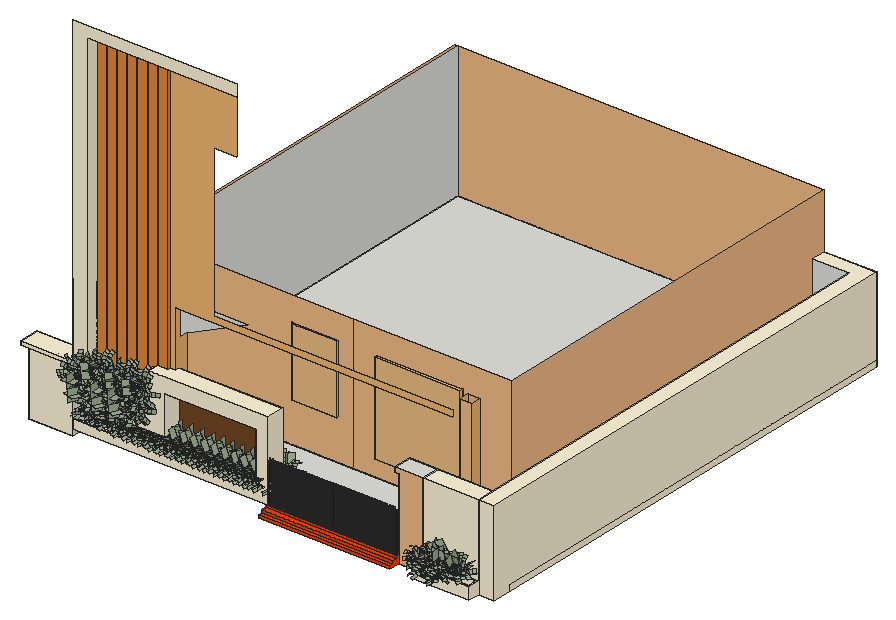
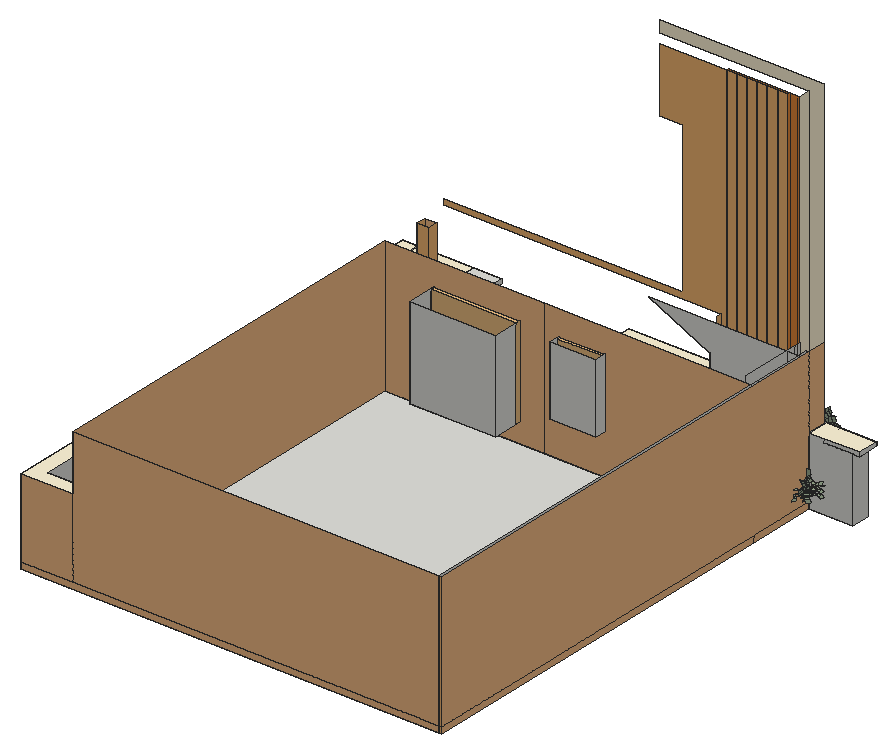
# SketchUp Ruby script. Lengths in inches.
U = 1.inch
M = Sketchup.active_model
def pt(a) = Geom::Point3d.new(a.map { |v| v * U })
def face(e, loops, mat)
  f = e.add_face(loops[0].map { |a| pt(a) })
  loops[1..].each { |l| e.add_face(l.map { |a| pt(a) }).erase! }
  f.material = f.back_material = mat if mat
  f
end
# faces: each face lists its corners as indices into pts; further lists are holes
def faces(e, pts, list, mat = nil) = list.each { |f| face(e, (f[0].is_a?(Array) ? f : [f]).map { |l| l.map { |i| pts[i] } }, mat) }
# xy, xz, yz: faces in a plane at the given z, y or x. An outline is a flat list of corners, or four numbers for a rectangle; further outlines are holes
def ring(l) = l.size == 4 ? [[l[0], l[1]], [l[2], l[1]], [l[2], l[3]], [l[0], l[3]]] : l.each_slice(2).to_a
def flat(e, list, mat, &to3) = list.each { |f| face(e, (f[0].is_a?(Array) ? f : [f]).map { |l| ring(l).map { |u, v| to3.(u, v) } }, mat) }
def xy(e, z, list, mat = nil) = flat(e, list, mat) { |x, y| [x, y, z] }
def xz(e, y, list, mat = nil) = flat(e, list, mat) { |x, z| [x, y, z] }
def yz(e, x, list, mat = nil) = flat(e, list, mat) { |y, z| [x, y, z] }
def lines(e, pts, list) = list.each { |a, b| e.add_line(pt(pts[a]), pt(pts[b])) }
# prism: a flat outline (further loops are holes) pulled along v
def prism(e, loops, v, mat = nil)
  f = face(e, loops, mat); d = Geom::Vector3d.new(v.map { |x| x * U })
  f.pushpull(f.normal.samedirection?(d) ? d.length : -d.length)
end
def box(e, o, s, mat = nil) = prism(e, [[o, [o[0] + s[0], o[1], o[2]], [o[0] + s[0], o[1] + s[1], o[2]], [o[0], o[1] + s[1], o[2]]]], [0, 0, s[2]], mat)
def at(x, y, z, deg = 0) = Geom::Transformation.translation(pt([x, y, z])) * Geom::Transformation.rotation(ORIGIN, Z_AXIS, deg.degrees)
def axes(o, x, y, z) = Geom::Transformation.new([*x, 0, *y, 0, *z, 0, *pt(o).to_a, 1])
def part(name) = M.definitions.add(name)
# library, detail: a bought-in or finely detailed component or shape, given as its bounding box
def library(name, o, s) = part(name).tap { |d| box(d.entities, o, s) }
def detail(e, o, s) = box(e.add_group.entities, o, s)
def put(e, d, t, mat = nil) = e.add_instance(d, t).tap { |i| i.material = mat if mat }
def group(e, t, mat = nil) = e.add_group.tap { |g| g.transformation = t; g.material = mat if mat }.entities
root = M.entities
M.materials.add("[Cladding Siding Tan]").color = [114, 71, 33]
M.materials.add("[Color B05]").color = [255, 63, 0]
M.materials.add("[Color C03]").color = [242, 183, 116]
M.materials.add("[Color C03]1").color = [242, 188, 135]
M.materials.add("[Color D01]").color = [255, 245, 216]
M.materials.add("[Color M08]").color = [30, 30, 30]
M.materials.add("[Wood Bamboo]").color = [226, 136, 59]
M.materials.add("hymenocallis littoralis").color = [156, 172, 146]
c1 = part("Group\#856")
xy(c1.entities,7.38,[[0,0,5.5,15.91]],"hymenocallis littoralis")
p = [[5.5,28.78,0],[5.5,26.79,3.44],[0,26.79,3.44],[0,28.78,0],[0,23.75,6],[5.5,23.75,6],
  [0,15.91,7.38],[5.5,15.91,7.38]]
faces(c1.entities,p,[[0,1,2,3],[4,2,1,5],[6,4,5,7]],"hymenocallis littoralis")
c2 = part("Group\#12")
xy(c2.entities,7.38,[[0,0,5.5,15.91],[0,15.91,5.5,23.87]],"hymenocallis littoralis")
p = [[5.5,31.07,4.3],[5.5,27.74,6.47],[0,27.74,6.47],[0,31.07,4.3],[0,23.87,7.38],[5.5,23.87,7.38]]
faces(c2.entities,p,[[0,1,2,3],[4,2,1,5]],"hymenocallis littoralis")
c3 = part("Group\#857")
xy(c3.entities,7.38,[[0,0,5.6,15.91]],"hymenocallis littoralis")
p = [[5.6,28.78,0],[5.6,26.79,3.44],[0,26.79,3.44],[0,28.78,0],[0,23.75,6],[5.6,23.75,6],
  [0,15.91,7.38],[5.6,15.91,7.38]]
faces(c3.entities,p,[[0,1,2,3],[4,2,1,5],[6,4,5,7]],"hymenocallis littoralis")
c4 = part("Group\#855")
put(c4.entities,c2,axes([6.09,8.57,-0.52],[0.446,0.85617,0.26089],[-0.18444,-0.19731,0.96283],[0.87582,-0.47754,0.0699]))
put(c4.entities,c2,axes([6.29,7.28,-1.71],[0.37058,0.92707,-0.05667],[-0.32382,0.19004,0.99128],[0.87712,-0.32925,0.34964]))
put(c4.entities,c2,axes([11.04,16.14,-0.7],[1,0,0],[0,0.16628,1.02662],[0,-1.18456,0.19186]))
c5 = part("Group\#860")
put(c5.entities,c1,axes([24.57,32.05,-1.76],[0.9552,-0.22102,-0.19681],[0.4036,0.95545,0.88585],[-0.00568,-0.67859,0.7345]))
put(c5.entities,c1,axes([23.95,29.24,-2.4],[0,1,0],[-0.76041,0,0.64945],[0.64945,0,0.76041]))
put(c5.entities,c1,axes([24.22,24.72,-0.48],[-0.70711,0.70711,0],[-0.32757,-0.32757,0.80237],[0.61237,0.61237,0.5]))
put(c5.entities,c2,axes([20.66,37.22,-0.63],[1.12361,0.03262,0.39091],[-0.43499,0.29739,0.78777],[0.09852,-1.27434,0.37535]))
put(c5.entities,c1,axes([28.75,24.45,-2.4],[-1,0,0],[0,-0.76041,0.64945],[0,0.64945,0.76041]))
put(c5.entities,c3,axes([30.4,30.98,-3.7],[0.65676,-0.72002,0.22414],[0.55667,0.66341,0.5],[-0.50871,-0.20361,0.83652]))
put(c5.entities,c3,axes([32.41,29.61,-3.7],[0.04029,-0.97372,0.22414],[0.85287,0.15038,0.5],[-0.52057,0.17102,0.83652]))
put(c5.entities,c1,axes([31.89,25.85,-1.76],[-0.92056,0.33739,-0.19681],[-0.5186,-0.89824,0.88585],[0.08952,0.67268,0.7345]))
put(c5.entities,c1,axes([25.55,34.78,-0.48],[0.86603,0.5,0],[-0.25,0.43301,0.86603],[0.43301,-0.75,0.5]))
put(c5.entities,c3,axes([20.4,16.9375,-8.07],[-0.70711,0.70711,0],[-0.35754,-0.35754,0.65422],[1.3987,1.3987,1.52882]))
put(c5.entities,c1,axes([32.86,34.14,-0.48],[0.76604,-0.64279,0],[0.32139,0.38302,0.86603],[-0.55667,-0.66341,0.5]))
put(c5.entities,c1,axes([27.15,34.7,-0.1],[0.82472,-0.17528,-0.53769],[0.53769,0.53769,0.64945],[0.17528,-0.82472,0.53769]))
put(c5.entities,c1,axes([33.58,28.77,-2.4],[0,-1,0],[0.76041,0,0.64945],[-0.64945,0,0.76041]))
put(c5.entities,c1,axes([26.43,23.87,-2.81],[-0.75126,0.04415,0.65853],[0.53769,-0.53769,0.64945],[0.38276,0.84199,0.3802]))
put(c5.entities,c1,axes([28.78,23.98,-2.4],[-1,0,0],[0,-0.76041,0.64945],[0,0.64945,0.76041]))
put(c5.entities,c1,axes([25.39,25.38,-2.4],[-0.70711,0.70711,0],[-0.53769,-0.53769,0.64945],[0.45923,0.45923,0.76041]))
put(c5.entities,c1,axes([27.32,21.63,-0.1],[-0.45923,0.70711,-0.53769],[-0.76041,0,0.64945],[0.45923,0.70711,0.53769]))
put(c5.entities,c1,axes([25.17,27.625,-1.76],[0.56416,0.80187,-0.19681],[-0.66673,0.66673,0.80532],[0.62659,-0.26057,0.7345]))
put(c5.entities,c3,axes([27.59,27.04,-3.96],[-0.8993,-0.06127,0.43301],[0.2962,-0.8138,0.5],[0.32175,0.57791,0.75]))
put(c5.entities,c3,axes([26.98,24.5,-3.18],[-0.5,0.86603,0],[-0.75,-0.43301,0.5],[0.43301,0.25,0.86603]))
put(c5.entities,c3,axes([24.55,27.74,-3.7],[0.29517,0.92878,0.22414],[-0.85287,0.15038,0.5],[0.43068,-0.33875,0.83652]))
put(c5.entities,c3,axes([24.26,29.8,-3.18],[0.76604,0.64279,0],[-0.47317,0.5639,0.425],[0.32139,-0.38302,0.86603]))
put(c5.entities,c3,axes([25.98,32.46,-3.18],[1,0,0],[0,0.86603,0.5],[0,-0.5,0.86603]))
put(c5.entities,c1,axes([28.78,33.57,-2.4],[1,0,0],[0,0.76041,0.64945],[0,-0.64945,0.76041]))
put(c5.entities,c4,at(14.99,21.38,2.5))
put(c5.entities,c2,axes([34.63,26.34,-1.46],[-0.70089,-0.70877,0.07994],[0.4756,-0.38088,0.79293],[-0.53156,0.59378,0.60405]))
put(c5.entities,c2,axes([28.14,16.92,1.8125],[-1.19719,0.6912,0],[-0.09607,-0.16641,0.94244],[0.68444,1.18549,0.17613]))
put(c5.entities,c2,axes([31.5625,35.84,0.97],[0.66765,-1.1564,0.35779],[0.04445,0.30732,0.91033],[-1.20828,-0.64496,0.17012]))
put(c5.entities,c2,axes([38.94,22.51,0.89],[-0.97932,-0.67164,-0.05202],[0.27787,-0.41401,0.90999],[-0.85985,0.93577,0.32097]))
put(c5.entities,c2,axes([38.44,21.09,1.98],[-1.02864,-0.54856,0.2395],[0.33481,0.06999,0.88388],[-0.77261,1.08328,0.06417]))
put(c5.entities,c3,axes([35.02,30.51,-1.3],[-0.17365,-0.98481,0],[0.60224,-0.10619,0.79122],[-0.7792,0.13739,0.61153]))
put(c5.entities,c3,axes([29.41,22.33,-1.3],[-0.93969,0.34202,0],[-0.20915,-0.57465,0.79122],[0.27061,0.74351,0.61153]))
put(c5.entities,c2,axes([19.64,36,-1.62],[1.18194,0.09546,0.08234],[-0.14377,0.68823,0.76313],[0.21457,-1.1326,0.62386]))
put(c5.entities,c3,axes([24.25,24.14,-1.3],[-0.34202,0.93969,0],[-0.57465,-0.20915,0.79122],[0.74351,0.27061,0.61153]))
put(c5.entities,c3,axes([25.98,34.61,-1.3],[1,0,0],[0,0.61153,0.79122],[0,-0.79122,0.61153]))
put(c5.entities,c3,axes([31.16,34.41,-1.64],[0.56518,-0.80224,-0.19234],[0.73413,0.34233,0.72935],[-0.47639,-0.50772,0.71782]))
put(c5.entities,c3,axes([40.52,26.84,-5.82],[-0.42262,-0.90631,0],[0.48019,-0.22391,0.68552],[-1.43418,0.66877,1.22305]))
put(c5.entities,c1,axes([29.86,38.42,-1.01],[0.89064,-0.37013,0.26413],[-0.03924,0.63286,1.01918],[-0.45353,-0.76487,0.45748]))
put(c5.entities,c1,axes([29.34,22.4,-0.48],[-0.99619,-0.08716,0],[0.04358,-0.4981,0.86603],[-0.07548,0.86273,0.5]))
c6 = part("Group\#859")
put(c6.entities,c1,axes([24.57,32.05,-1.76],[0.9552,-0.22102,-0.19681],[0.4036,0.95545,0.88585],[-0.00568,-0.67859,0.7345]))
put(c6.entities,c1,axes([23.95,29.24,-2.4],[0,1,0],[-0.76041,0,0.64945],[0.64945,0,0.76041]))
put(c6.entities,c1,axes([24.22,24.72,-0.48],[-0.70711,0.70711,0],[-0.32757,-0.32757,0.80237],[0.61237,0.61237,0.5]))
put(c6.entities,c2,axes([22.87,39.97,-0.63],[1.12361,0.03262,0.39091],[-0.43499,0.29739,0.78777],[0.09852,-1.27434,0.37535]))
put(c6.entities,c1,axes([28.75,24.45,-2.4],[-1,0,0],[0,-0.76041,0.64945],[0,0.64945,0.76041]))
put(c6.entities,c3,axes([30.4,30.98,-3.7],[0.65676,-0.72002,0.22414],[0.55667,0.66341,0.5],[-0.50871,-0.20361,0.83652]))
put(c6.entities,c3,axes([32.41,29.61,-3.7],[0.04029,-0.97372,0.22414],[0.85287,0.15038,0.5],[-0.52057,0.17102,0.83652]))
put(c6.entities,c1,axes([31.89,25.85,-1.76],[-0.92056,0.33739,-0.19681],[-0.5186,-0.89824,0.88585],[0.08952,0.67268,0.7345]))
put(c6.entities,c1,axes([25.55,34.78,-0.48],[0.86603,0.5,0],[-0.25,0.43301,0.86603],[0.43301,-0.75,0.5]))
put(c6.entities,c3,axes([20.4,16.9375,-8.07],[-0.70711,0.70711,0],[-0.35754,-0.35754,0.65422],[1.3987,1.3987,1.52882]))
put(c6.entities,c1,axes([32.86,34.14,-0.48],[0.76604,-0.64279,0],[0.32139,0.38302,0.86603],[-0.55667,-0.66341,0.5]))
put(c6.entities,c1,axes([27.15,34.7,-0.1],[0.82472,-0.17528,-0.53769],[0.53769,0.53769,0.64945],[0.17528,-0.82472,0.53769]))
put(c6.entities,c1,axes([33.58,28.77,-2.4],[0,-1,0],[0.76041,0,0.64945],[-0.64945,0,0.76041]))
put(c6.entities,c1,axes([26.43,23.87,-2.81],[-0.75126,0.04415,0.65853],[0.53769,-0.53769,0.64945],[0.38276,0.84199,0.3802]))
put(c6.entities,c1,axes([28.78,23.98,-2.4],[-1,0,0],[0,-0.76041,0.64945],[0,0.64945,0.76041]))
put(c6.entities,c1,axes([25.39,25.38,-2.4],[-0.70711,0.70711,0],[-0.53769,-0.53769,0.64945],[0.45923,0.45923,0.76041]))
put(c6.entities,c1,axes([27.32,21.63,-0.1],[-0.45923,0.70711,-0.53769],[-0.76041,0,0.64945],[0.45923,0.70711,0.53769]))
put(c6.entities,c1,axes([25.17,27.625,-1.76],[0.56416,0.80187,-0.19681],[-0.66673,0.66673,0.80532],[0.62659,-0.26057,0.7345]))
put(c6.entities,c3,axes([27.59,27.04,-3.96],[-0.8993,-0.06127,0.43301],[0.2962,-0.8138,0.5],[0.32175,0.57791,0.75]))
put(c6.entities,c3,axes([33.07,28.9375,-1.86],[-0.5,0.86603,0],[-0.86347,-0.49852,0.1661],[0.11853,0.06843,0.98016]))
put(c6.entities,c3,axes([24.55,27.74,-3.7],[0.29517,0.92878,0.22414],[-0.85287,0.15038,0.5],[0.43068,-0.33875,0.83652]))
put(c6.entities,c3,axes([24.26,29.8,-3.18],[0.76604,0.64279,0],[-0.47317,0.5639,0.425],[0.32139,-0.38302,0.86603]))
put(c6.entities,c3,axes([25.98,32.46,-3.18],[1,0,0],[0,0.86603,0.5],[0,-0.5,0.86603]))
put(c6.entities,c1,axes([28.78,33.57,-2.4],[1,0,0],[0,0.76041,0.64945],[0,-0.64945,0.76041]))
put(c6.entities,c4,at(14.99,21.38,2.5))
put(c6.entities,c2,axes([34.63,26.34,-1.46],[-0.70089,-0.70877,0.07994],[0.4756,-0.38088,0.79293],[-0.53156,0.59378,0.60405]))
put(c6.entities,c2,axes([28.14,16.92,1.8125],[-1.19719,0.6912,0],[-0.09607,-0.16641,0.94244],[0.68444,1.18549,0.17613]))
put(c6.entities,c2,axes([31.5625,35.84,0.97],[0.66765,-1.1564,0.35779],[0.04445,0.30732,0.91033],[-1.20828,-0.64496,0.17012]))
put(c6.entities,c2,axes([38.94,22.51,0.89],[-0.97932,-0.67164,-0.05202],[0.27787,-0.41401,0.90999],[-0.85985,0.93577,0.32097]))
put(c6.entities,c2,axes([38.44,21.09,1.98],[-1.02864,-0.54856,0.2395],[0.33481,0.06999,0.88388],[-0.77261,1.08328,0.06417]))
put(c6.entities,c3,axes([35.02,30.51,-1.3],[-0.17365,-0.98481,0],[0.60224,-0.10619,0.79122],[-0.7792,0.13739,0.61153]))
put(c6.entities,c3,axes([29.41,22.33,-1.3],[-0.93969,0.34202,0],[-0.20915,-0.57465,0.79122],[0.27061,0.74351,0.61153]))
put(c6.entities,c2,axes([19.64,36,-1.62],[1.18194,0.09546,0.08234],[-0.14377,0.68823,0.76313],[0.21457,-1.1326,0.62386]))
put(c6.entities,c3,axes([24.25,24.14,-1.3],[-0.34202,0.93969,0],[-0.57465,-0.20915,0.79122],[0.74351,0.27061,0.61153]))
put(c6.entities,c3,axes([25.98,34.61,-1.3],[1,0,0],[0,0.61153,0.79122],[0,-0.79122,0.61153]))
put(c6.entities,c3,axes([31.16,34.41,-1.64],[0.56518,-0.80224,-0.19234],[0.73413,0.34233,0.72935],[-0.47639,-0.50772,0.71782]))
put(c6.entities,c3,axes([40.52,26.84,-5.82],[-0.42262,-0.90631,0],[0.48019,-0.22391,0.68552],[-1.43418,0.66877,1.22305]))
put(c6.entities,c1,axes([29.86,38.42,-1.01],[0.89064,-0.37013,0.26413],[-0.03924,0.63286,1.01918],[-0.45353,-0.76487,0.45748]))
put(c6.entities,c1,axes([29.34,22.4,-0.48],[-0.99619,-0.08716,0],[0.04358,-0.4981,0.86603],[-0.07548,0.86273,0.5]))
put(c6.entities,c3,axes([25.22,28.39,-0.16],[0.48481,0.87462,0],[-0.87203,0.48338,0.1661],[0.11971,-0.06635,0.98016]))
put(c6.entities,c3,axes([24.56,24.29,-4.78],[0.48481,0.87462,0],[-0.87203,0.48338,0.1661],[0.11971,-0.06635,0.98016]))
put(c6.entities,c3,axes([23.9375,27.06,-4.78],[0.99753,0.07018,0],[-0.06998,0.99459,0.1661],[0.00961,-0.13653,0.98016]))
put(c6.entities,c3,axes([25.92,29.09,-4.78],[0.6025,-0.79812,0],[0.79576,0.60072,0.1661],[-0.10924,-0.08246,0.98016]))
put(c6.entities,c3,axes([28.7,28.53,-4.78],[-0.34082,-0.94013,0],[0.93735,-0.33981,0.1661],[-0.12867,0.04665,0.98016]))
c7 = part("Group\#858")
xz(c7.entities,10.07,[[9.07,0,10.07,31.01],[0,31.01,0,45.12,20.13,45.12,20.13,31.01,10.07,31.01,10.07,32.58,9.07,32.58,9.07,31.01]],"hymenocallis littoralis")
yz(c7.entities,10.07,[[0,31.01,20.13,45.12]],"hymenocallis littoralis")
p = [[9.57,9.2,0],[10.07,10.07,0],[10.07,10.07,31.01],[10.07,10.07,32.58],[9.57,9.2,32.58]]
faces(c7.entities,p,[[0,1,2,3,4]],"hymenocallis littoralis")
c8 = part("cây lá nắng")
put(c8.entities,c5,axes([49.26,-2.75,0],[0.63109,0.63109,0],[-0.63109,0.63109,0],[0,0,0.935]))
put(c8.entities,c6,axes([26.6,-8.68,0],[0.63109,0.63109,0],[-0.63109,0.63109,0],[0,0,0.935]))
put(c8.entities,c7,axes([29.71,14.29,6.94],[0.425,0.73612,0],[-0.6771,0.39092,-0.33349],[-0.26859,0.15507,0.72712]))
put(c8.entities,c7,axes([42.0625,26.12,6.94],[0.85,0,0],[0,0.78185,-0.33349],[0,0.33349,0.78185]))
put(c8.entities,c5,axes([7.3125,23.0625,0],[0.8925,0,0],[0,0.8925,0],[0,0,0.935]))
put(c8.entities,c7,axes([24.4375,40.23,2.05],[0.85,0,0],[0,0.85,0],[0,0,0.85]))
c9 = part("Planting+101")
put(c9.entities,c8,axes([21.34,32.96,-4.59],[0,-0.71,0],[-0.71,0,0],[0,0,0.71]))
c10 = part("Group\#428")
prism(c10.entities,[[[0,1.97,0],[0,1.97,1.18],[0,0,1.18],[0,0,0]],[[0,1.92,1.13],[0,1.92,0.05],[0,0.05,0.05],[0,0.05,1.13]]],[98.43,0,0])
c11 = part("Group\#430")
xy(c11.entities,0,[[0.3,0,0.22,0.01,0.15,0.04,0.09,0.09,0.04,0.15,0.01,0.22,0,0.3,0.3,0.3],[0.3,0,0.3,0.3,0.59,0.3,0.58,0.22,0.55,0.15,0.5,0.09,0.44,0.04,0.37,0.01],[0,0.3,0.01,0.37,0.04,0.44,0.09,0.5,0.15,0.55,0.22,0.58,0.3,0.59,0.3,0.3],[0.3,0.3,0.3,0.59,0.37,0.58,0.44,0.55,0.5,0.5,0.55,0.44,0.58,0.37,0.59,0.3]])
xy(c11.entities,39.37,[[0.3,0,0.37,0.01,0.44,0.04,0.5,0.09,0.55,0.15,0.58,0.22,0.59,0.3,0.58,0.37,0.55,0.44,0.5,0.5,0.44,0.55,0.37,0.58,0.3,0.59,0.22,0.58,0.15,0.55,0.09,0.5,0.04,0.44,0.01,0.37,0,0.3,0.01,0.22,0.04,0.15,0.09,0.09,0.15,0.04,0.22,0.01]])
p = [[0.09,0.09,0],[0.15,0.04,0],[0.15,0.04,39.37],[0.09,0.09,39.37],[0.22,0.01,0],[0.22,0.01,39.37],
  [0.3,0,0],[0.3,0,39.37],[0.37,0.01,0],[0.37,0.01,39.37],[0.44,0.04,0],[0.44,0.04,39.37],
  [0.5,0.09,0],[0.5,0.09,39.37],[0.01,0.22,0],[0.04,0.15,0],[0.04,0.15,39.37],[0.01,0.22,39.37],
  [0.55,0.15,0],[0.55,0.15,39.37],[0.58,0.22,0],[0.58,0.22,39.37],[0,0.3,0],[0,0.3,39.37],
  [0.59,0.3,0],[0.59,0.3,39.37],[0.01,0.37,0],[0.01,0.37,39.37],[0.58,0.37,0],[0.58,0.37,39.37],
  [0.09,0.5,0],[0.04,0.44,0],[0.04,0.44,39.37],[0.09,0.5,39.37],[0.55,0.44,0],[0.5,0.5,0],
  [0.5,0.5,39.37],[0.55,0.44,39.37],[0.15,0.55,0],[0.15,0.55,39.37],[0.44,0.55,0],[0.44,0.55,39.37],
  [0.22,0.58,0],[0.22,0.58,39.37],[0.3,0.59,0],[0.3,0.59,39.37],[0.37,0.58,0],[0.37,0.58,39.37]]
faces(c11.entities,p,[[0,1,2,3],[1,4,5,2],[4,6,7,5],[6,8,9,7],[8,10,11,9],[10,12,13,11],[14,15,16,17],[15,0,3,16],
  [12,18,19,13],[18,20,21,19],[22,14,17,23],[20,24,25,21],[26,22,23,27],[24,28,29,25],[30,31,32,33],[31,26,27,32],
  [34,35,36,37],[28,34,37,29],[38,30,33,39],[35,40,41,36],[42,38,39,43],[44,42,43,45],[46,44,45,47],[40,46,47,41]])
c12 = part("Group\#429")
prism(c12.entities,[[[0.01,0.22,35.83],[0,0.3,35.83],[0.01,0.37,35.83],[0.04,0.44,35.83],[0.09,0.5,35.83],[0.15,0.55,35.83],[0.22,0.58,35.83],[0.3,0.59,35.83],[0.37,0.58,35.83],[0.44,0.55,35.83],[0.5,0.5,35.83],[0.55,0.44,35.83],[0.58,0.37,35.83],[0.59,0.3,35.83],[0.58,0.22,35.83],[0.55,0.15,35.83],[0.5,0.09,35.83],[0.44,0.04,35.83],[0.37,0.01,35.83],[0.3,0,35.83],[0.22,0.01,35.83],[0.15,0.04,35.83],[0.09,0.09,35.83],[0.04,0.15,35.83]]],[0,0,3.54])
c13 = part("Picket railing panel")
g1 = group(c13.entities,at(0,0,0))
put(g1,c10,axes([0,0,39.76],[1,0,0],[0,0,-1],[0,1,0]),"[Color M08]")
put(g1,c10,axes([0,0,1.97],[1,0,0],[0,0,-1],[0,1,0]),"[Color M08]")
put(g1,c10,axes([98.43,0,37.8],[0,0,-0.364],[-1,0,0],[0,1,0]),"[Color M08]")
put(g1,c10,axes([1.97,0,37.8],[0,0,-0.364],[-1,0,0],[0,1,0]),"[Color M08]")
g2 = group(c13.entities,at(1.67,0.3,1.97))
put(g2,c11,at(78.74,0,0),"[Color M08]")
put(g2,c11,at(90.55,0,0),"[Color M08]")
put(g2,c11,at(82.68,0,0),"[Color M08]")
put(g2,c11,at(86.61,0,0),"[Color M08]")
put(g2,c11,at(66.93,0,0),"[Color M08]")
put(g2,c11,at(11.8125,0,0),"[Color M08]")
put(g2,c11,at(15.75,0,0),"[Color M08]")
put(g2,c11,at(47.24,0,0),"[Color M08]")
put(g2,c11,at(59.06,0,0),"[Color M08]")
put(g2,c12,at(0,0,0),"[Color M08]")
put(g2,c11,at(39.37,0,0),"[Color M08]")
put(g2,c11,at(62.99,0,0),"[Color M08]")
put(g2,c11,at(55.12,0,0),"[Color M08]")
put(g2,c11,at(19.69,0,0),"[Color M08]")
put(g2,c11,at(35.43,0,0),"[Color M08]")
put(g2,c11,at(7.875,0,0),"[Color M08]")
put(g2,c11,at(23.62,0,0),"[Color M08]")
put(g2,c11,at(31.5,0,0),"[Color M08]")
put(g2,c11,at(43.31,0,0),"[Color M08]")
put(g2,c11,at(27.56,0,0),"[Color M08]")
put(g2,c11,at(3.9375,0,0),"[Color M08]")
put(g2,c11,at(51.18,0,0),"[Color M08]")
put(g2,c11,at(70.87,0,0),"[Color M08]")
put(g2,c11,at(74.8,0,0),"[Color M08]")
put(g2,c12,at(94.49,0,0),"[Color M08]")
c14 = library("Group\#5",[0,0,0],[84,7.18,89.375])
c15 = part("Group\#3")
yz(c15.entities,10,[[0,0,3,309.43]])
g3 = group(c15.entities,at(0,0,0))
xz(g3,0,[[0,0,10,309.43]])
c16 = library("French glass door with glass lintels",[-8.63,0,-6],[91.05,103.25,8])
c17 = library("0bf58b33-bf0e-48eb-9a0e-7b561c723b43",[30.51,1.97,38.58],[7.49,3.24,2.84])
c18 = library("53c5b651-04ed-452e-9df6-41195152b95b",[21.06,1.97,38.58],[7.48,3.24,2.84])
xy(root,0,[[241.3125,20.4,241.3125,49.9,52.3125,49.9,52.3125,117.47,412.3125,117.47,412.3125,49.9,370.28,49.9,370.28,20.4],[393.97,20.4,448.3125,49.9],[6.375,31.9,49.3125,49.9],[370.28,31.9,393.97,49.9],[448.3125,31.9,463.8125,49.9],
  [49.3125,49.9,52.3125,117.47],[412.3125,49.9,412.3125,117.47,52.3125,117.47,52.3125,501.47,463.8125,501.47,463.8125,49.9],[49.3125,117.47,52.3125,501.47]])
xy(root,2.66,[[241.3125,20.4,370.28,24.71]],"[Color B05]")
xy(root,4.375,[[395.18,21.61,447.1,30.69]],"[Color D01]")
xy(root,5.3125,[[241.3125,24.71,370.28,29.52]],"[Color B05]")
xy(root,6,[[49.3125,31.9,241.3125,49.9],[[241.3125,31.9,370.28,31.9,370.28,49.9,448.3125,49.9,448.3125,486.84,412.3125,486.84,412.3125,117.47,52.3125,117.47,52.3125,109.47,63.88,109.47,63.88,59.47,229.04,59.47,229.04,49.9,241.3125,49.9],[399.28,70.78,410.47,80.47]],[49.3125,49.9,52.3125,59.47],[52.3125,49.9,63.88,59.47],[63.88,49.9,139.52,59.47],
  [139.52,49.9,199.52,59.47],[199.52,49.9,229.04,59.47],[448.3125,49.9,463.8125,49.9,463.8125,501.47,412.3125,501.47,412.3125,486.84,448.3125,486.84],[49.3125,59.47,52.3125,109.47],[52.3125,59.47,63.88,109.47],
  [49.3125,109.47,52.3125,117.47],[49.3125,117.47,52.3125,501.47],[52.3125,117.47,412.3125,501.47]])
xy(root,7.3125,[[241.3125,29.52,370.28,31.9]],"[Color B05]")
xy(root,7.8,[[52.05,34.64,226.3,47.16]])
xy(root,12,[[[393.97,20.4,448.3125,31.9],[395.18,21.61,447.1,30.69]]],"[Color D01]")
xy(root,14.3,[[[49.3125,31.9,229.04,49.9],[52.05,34.64,226.3,47.16]]],"[Color D01]")
xy(root,24.625,[[280.3125,117.47,364.3125,146.78]])
xy(root,30.5625,[[49.3125,31.9,139.52,49.9]])
xy(root,45.57,[[63.88,42.9,73.88,42.9,73.88,45.9,123.75,45.9,123.75,49.9,63.88,49.9]])
xy(root,45.57,[[63.88,31.9,123.75,31.9,123.75,45.9,73.88,45.9,73.88,42.9,63.88,42.9]],"[Color D01]")
xy(root,46.125,[[196.3125,117.47,241.3125,128.9]])
xy(root,63.39,[[0,29.15,34.8125,31.9],[34.8125,29.15,49.3125,31.9],[0,31.9,6.375,49.9],[6.375,31.9,34.8125,49.9]])
xy(root,67.02,[[0,29.15,49.3125,49.9]],"[Color D01]")
xy(root,68.78,[[139.52,31.9,229.04,49.9],[139.52,49.9,229.04,59.47]])
xy(root,79.13,[[366.09,31.9,370.28,49.9]])
xy(root,83.44,[[366.09,31.9,393.97,49.9],[123.75,45.9,139.52,49.9]])
xy(root,83.44,[[123.75,31.9,241.3125,31.9,241.3125,49.9,139.52,49.9,139.52,45.9,123.75,45.9],[393.97,31.9,448.3125,49.9],[448.3125,31.9,463.8125,31.9,463.8125,501.47,412.3125,501.47,412.3125,486.84,448.3125,486.84]],"[Color D01]")
xz(root,20.4,[[241.3125,0,370.28,2.66]],"[Color B05]")
xz(root,20.4,[[393.97,0,448.3125,12]],"[Color D01]")
xz(root,21.61,[[395.18,4.375,447.1,12]],"[Color D01]")
xz(root,24.71,[[241.3125,2.66,370.28,5.3125]],"[Color B05]")
xz(root,29.15,[[0,63.39,49.3125,67.02]],"[Color D01]")
xz(root,29.52,[[241.3125,5.3125,370.28,7.3125]],"[Color B05]")
xz(root,30.69,[[395.18,4.375,447.1,12]],"[Color D01]")
xz(root,31.9,[[241.3125,6,370.28,7.3125]])
xz(root,31.9,[[370.28,0,393.97,0,393.97,83.44,366.09,83.44,366.09,79.13,370.28,79.13]],"[Color C03]1")
xz(root,31.9,[[6.375,0,49.3125,63.39],[448.3125,0,463.8125,83.44],[49.3125,6,241.3125,6,241.3125,83.44,123.75,83.44,123.75,45.57,63.88,45.57,63.88,354.99,210.46,354.99,210.46,366,49.3125,366,49.3125,30.5625,139.52,30.5625,139.52,68.78,229.04,68.78,229.04,14.3,49.3125,14.3],[393.97,12,448.3125,83.44]],"[Color D01]")
xz(root,34.64,[[52.05,7.8,226.3,14.3]])
xz(root,45.9,[[73.88,45.57,123.75,45.57,123.75,83.44,139.52,83.44,139.52,138,412.3125,138,412.3125,144,177.125,144,177.125,291.78,199.52,291.78,199.52,354.99,73.88,354.99]],"[Color C03]")
xz(root,47.16,[[52.05,7.8,52.3125,14.3],[52.3125,7.8,63.88,14.3],[63.88,7.8,226.3,14.3]])
xz(root,49.9,[[6.375,0,6.375,63.39,34.8125,63.39,34.8125,67.02,49.3125,67.02,49.3125,0],[49.3125,0,52.3125,6],[370.28,0,393.97,6],[393.97,0,448.3125,6],[448.3125,0,463.8125,6],
  [49.3125,6,52.3125,14.3],[52.3125,6,63.88,14.3],[63.88,6,229.04,14.3],[229.04,6,229.04,68.78,139.52,68.78,139.52,83.44,241.3125,83.44,241.3125,6],[370.28,6,370.28,79.13,366.09,79.13,366.09,83.44,393.97,83.44,393.97,6],
  [393.97,6,448.3125,83.44],[49.3125,30.5625,52.3125,138],[63.88,30.5625,123.75,45.57],[123.75,30.5625,139.52,83.44],[0,63.39,34.8125,67.02]])
xz(root,49.9,[[49.3125,14.3,52.3125,30.5625],[52.3125,14.3,63.88,30.5625],[63.88,14.3,229.04,14.3,229.04,68.78,139.52,68.78,139.52,30.5625,63.88,30.5625]],"[Cladding Siding Tan]")
xz(root,49.9,[[52.3125,0,241.3125,6]],"[Color D01]")
xz(root,59.47,[[52.3125,6,52.3125,138,199.52,138,139.52,109.96,139.52,68.78,229.04,68.78,229.04,6]])
xz(root,70.78,[[399.28,6,410.47,138]],"[Color C03]1")
xz(root,80.47,[[399.28,6,410.47,138]],"[Color C03]")
xz(root,117.47,[[49.3125,0,52.3125,6],[52.3125,0,412.3125,6]])
xz(root,117.47,[[[52.3125,6,256.62,138],[196.3125,46.125,241.3125,114]],[[256.62,6,412.3125,138],[280.3125,24.625,364.3125,114]]],"[Color C03]1")
xz(root,128.9,[[196.3125,46.125,241.3125,114]])
xz(root,146.78,[[280.3125,24.625,364.3125,114]])
xz(root,486.84,[[412.3125,6,448.3125,83.44]])
xz(root,501.47,[[49.3125,0,52.3125,6],[49.3125,6,52.3125,138]],"[Color C03]")
xz(root,501.47,[[52.3125,0,463.8125,6],[52.3125,6,412.3125,138],[412.3125,6,463.8125,83.44]],"[Color C03]1")
yz(root,0,[[29.15,63.39,49.9,67.02]])
yz(root,6.375,[[31.9,0,49.9,63.39]])
yz(root,49.3125,[[31.9,0,49.9,6],[31.9,6,49.9,14.3],[31.9,14.3,49.9,30.5625],[31.9,30.5625,49.9,67.02],[29.15,63.39,31.9,67.02]])
yz(root,49.3125,[[49.9,0,117.47,6],[117.47,0,501.47,6],[49.9,6,501.47,138],[31.9,67.02,49.9,138]],"[Color C03]1")
yz(root,52.05,[[34.64,7.8,47.16,14.3]])
yz(root,52.3125,[[49.9,0,117.47,6],[117.47,0,501.47,6],[49.9,6,59.47,138],[59.47,6,109.47,138],[109.47,6,117.47,138],
  [117.47,6,501.47,138]])
yz(root,63.88,[[49.9,6,109.47,138],[42.9,45.57,49.9,138]])
yz(root,63.88,[[31.9,45.57,42.9,354.99]],"[Color D01]")
yz(root,123.75,[[31.9,45.57,45.9,83.44],[45.9,45.57,49.9,83.44]])
yz(root,139.52,[[49.9,68.78,59.47,68.78,59.47,109.96,50.65,109.96,50.65,138,45.9,138,45.9,83.44,49.9,83.44]],"[Color C03]")
yz(root,139.52,[[31.9,30.5625,49.9,68.78]],"[Color D01]")
yz(root,196.3125,[[117.47,46.125,128.9,114]])
yz(root,226.3,[[34.64,7.8,47.16,14.3]])
yz(root,229.04,[[49.9,6,59.47,68.78]])
yz(root,229.04,[[31.9,14.3,49.9,68.78]],"[Color D01]")
yz(root,241.3125,[[117.47,46.125,128.9,114]])
yz(root,241.3125,[[20.4,0,20.4,2.66,24.71,2.66,24.71,5.3125,29.52,5.3125,29.52,7.3125,31.9,7.3125,31.9,6,49.9,6,49.9,0]],"[Color B05]")
yz(root,241.3125,[[31.9,6,49.9,83.44]],"[Color D01]")
yz(root,280.3125,[[117.47,24.625,146.78,114]])
yz(root,364.3125,[[117.47,24.625,146.78,114]])
yz(root,366.09,[[31.9,79.13,49.9,83.44]])
yz(root,370.28,[[31.9,0,49.9,6],[31.9,6,49.9,79.13]])
yz(root,370.28,[[20.4,0,31.9,0,31.9,7.3125,29.52,7.3125,29.52,5.3125,24.71,5.3125,24.71,2.66,20.4,2.66]],"[Color B05]")
yz(root,393.97,[[31.9,0,49.9,83.44]])
yz(root,393.97,[[20.4,0,31.9,12]],"[Color D01]")
yz(root,395.18,[[21.61,4.375,30.69,12]],"[Color D01]")
yz(root,399.28,[[70.78,6,80.47,138]],"[Color C03]")
yz(root,410.47,[[70.78,6,80.47,138]],"[Color C03]")
yz(root,412.3125,[[117.47,6,486.84,6,486.84,83.44,501.47,83.44,501.47,138,117.47,138]],"[Color C03]1")
yz(root,447.1,[[21.61,4.375,30.69,12]],"[Color D01]")
yz(root,448.3125,[[31.9,0,49.9,83.44],[49.9,6,486.84,83.44]])
yz(root,448.3125,[[20.4,0,31.9,12]],"[Color D01]")
yz(root,463.8125,[[31.9,0,49.9,0,49.9,6,501.47,6,501.47,83.44,31.9,83.44],[49.9,0,501.47,6]],"[Color D01]")
p = [[34.8125,31.9,67.02],[34.8125,31.9,63.39]]
lines(root,p,[[0,1]])
put(root,c5,axes([418,50.4375,1.34],[0,-0.63368,0],[-0.63368,0,0],[0,0,0.66385]))
put(root,c6,axes([440.54,36.75,1.34],[-0.44808,-0.44808,0],[-0.44808,0.44808,0],[0,0,0.66385]))
put(root,c3,axes([419.6,19.1,-4.02],[0,0.63367,0],[0.32041,0,0.43431],[-1.25345,0,1.01491]))
put(root,c3,axes([406.15,14.53,-2.52],[0.59546,-0.21673,0],[-0.11483,-0.31549,0.45508],[0.34296,0.94228,0.81192]))
put(root,c3,axes([411.85,20.41,-1.29],[0.43041,0.3755,0.28746],[0.23192,-0.49736,0.33192],[-0.40311,0.11478,0.49789]))
put(root,c3,axes([408.82,20.92,-1.12],[0.02834,-0.6169,0.1488],[-0.54669,0.04783,0.33192],[0.31917,0.13671,0.55532]))
put(root,c3,axes([408.54,19.4,-1.12],[0.41825,-0.45435,0.1488],[-0.44953,-0.31477,0.33192],[0.15662,0.30988,0.55532]))
put(root,c3,axes([410.14,23.56,-0.77],[-0.44808,-0.44808,0],[-0.38805,0.38805,0.33192],[0.22404,-0.22404,0.57491]))
put(root,c3,axes([412.1,23.14,-0.77],[-0.63126,-0.05523,0],[-0.04065,0.46469,0.28214],[0.02761,-0.31563,0.57491]))
put(root,c3,axes([413.26,19.54,-0.77],[-0.16401,0.61208,0],[0.53008,0.14203,0.33192],[-0.30604,-0.082,0.57491]))
put(root,c1,axes([414.39,18.1,1.27],[-0.11107,0.52261,-0.35694],[0.34072,0.34072,0.43114],[-0.52261,0.11107,0.35694]))
put(root,c1,axes([410.46,17.95,0.17],[0.2613,0.56366,-0.13065],[0.63485,-0.17011,0.58807],[-0.34152,0.2613,0.4876]))
put(root,c1,axes([412.49,23.03,-0.26],[-0.44808,0.44808,0],[0.34072,0.34072,0.43114],[-0.291,-0.291,0.5048]))
put(root,c1,axes([412.49,18.73,-0.26],[0.44808,0.44808,0],[0.34072,-0.34072,0.43114],[-0.291,0.291,0.5048]))
put(root,c1,axes([412.69,18.5,-0.26],[0.44808,0.44808,0],[0.34072,-0.34072,0.43114],[-0.291,0.291,0.5048]))
put(root,c1,axes([413.58,20.65,-0.26],[0,0.63367,0],[0.48185,0,0.43114],[-0.41154,0,0.5048]))
put(root,c3,axes([409.18,24.52,0.47],[-0.44808,-0.44808,0],[-0.27401,0.27401,0.52525],[0.35453,-0.35453,0.40596]))
put(root,c3,axes([406.97,18.64,0.47],[0.51908,-0.36346,0],[-0.22227,-0.31743,0.52525],[0.28758,0.41071,0.40596]))
put(root,c3,axes([413.15,17.48,0.47],[0.2678,0.5743,0],[0.3512,-0.16377,0.52525],[-0.4544,0.21189,0.40596]))
put(root,c3,axes([414.65,20.61,0.47],[-0.2678,0.5743,0],[0.3512,0.16377,0.52525],[-0.4544,-0.21189,0.40596]))
put(root,c1,axes([405.73,24.49,0.67],[-0.23323,-0.56492,0.17534],[-0.26598,0.30115,0.67658],[0.54593,-0.1395,0.3037]))
put(root,c1,axes([409.3,24.79,1.02],[-0.61208,-0.16401,0],[-0.082,0.30604,0.57491],[0.14203,-0.53008,0.33193]))
put(root,c1,axes([413.15,17.55,1.02],[0.48542,0.40732,0],[0.20366,-0.24271,0.57491],[-0.35275,0.42039,0.33193]))
put(root,c1,axes([414.4,20.88,1.02],[0,0.63367,0],[0.29355,0,0.53266],[-0.54878,0,0.33193]))
put(root,c7,axes([415.84,25.77,6.26],[0,-0.6035,0],[-0.55511,0,-0.23678],[-0.23678,0,0.55511]))
put(root,c7,axes([424.23,34.54,6.26],[-0.52265,-0.30175,0],[-0.27756,0.48074,-0.23678],[-0.1101,0.1907,0.51625]))
put(root,c2,axes([410.4,28.07,0.92],[-0.51808,-0.48885,0.25951],[0.06166,0.32816,0.52296],[0.52686,-0.61515,0.24917]))
put(root,c2,axes([411.4,27.98,0.26],[-0.57237,-0.48683,0.05466],[-0.24396,0.3728,0.5066],[0.41135,-0.60363,0.41415]))
put(root,c2,axes([409.01,16.9375,0.36],[0.63164,-0.00353,0.05307],[-0.04244,-0.38377,0.52639],[-0.02788,0.50424,0.401]))
put(root,c2,axes([406.125,22.57,1.98],[0.219,-0.81731,0.23752],[-0.15762,0.11779,0.60432],[0.83039,0.25241,0.11294]))
put(root,c4,axes([420.03,23.52,2.99],[-0.44808,-0.44808,0],[-0.44808,0.44808,0],[0,0,0.66385]))
put(root,c7,axes([405.82,38.28,2.79],[0,-0.6035,0],[-0.6035,0,0],[0,0,0.6035]))
put(root,c9,at(88.79,42.42,14.3))
put(root,c9,at(102.36,42.42,14.3))
put(root,c9,at(113.04,42.42,14.3))
put(root,c9,at(123.73,42.42,14.3))
put(root,c9,at(134.42,42.42,14.3))
put(root,c9,at(145.11,42.42,14.3))
put(root,c9,at(155.79,42.42,14.3))
put(root,c9,at(166.48,42.42,14.3))
put(root,c9,at(177.17,42.42,14.3))
put(root,c9,at(187.86,42.42,14.3))
put(root,c9,at(197.48,42.42,14.3))
put(root,c9,at(207.11,42.42,14.3))
put(root,c9,at(216.73,42.42,14.3))
put(root,c9,at(226.36,42.42,14.3))
put(root,c9,at(235.98,42.42,14.3))
put(root,c9,at(63.88,45.16,14.3))
put(root,c5,axes([389.3,37.74,10.02],[0.63368,0,0],[0,-0.63368,0],[0,0,0.66385]))
put(root,c5,axes([404.18,37.74,10.02],[0.63368,0,0],[0,-0.63368,0],[0,0,0.66385]))
put(root,c5,axes([433.96,50.875,10.02],[0.44808,-0.44808,0],[-0.44808,-0.44808,0],[0,0,0.66385]))
put(root,c6,axes([417.87,55.09,10.02],[0.44808,-0.44808,0],[-0.44808,-0.44808,0],[0,0,0.66385]))
put(root,c13,axes([241.3125,31.9,6],[0.645,0,0],[0,1,0],[0,0,1]))
put(root,c13,axes([303.25,31.9,6],[0.645,0,0],[0,1,0],[0,0,1]))
put(root,c7,axes([428.85,30.38,14.95],[0.6035,0,0],[0,-0.55511,-0.23678],[0,-0.23678,0.55511]))
put(root,c7,axes([420.08,38.78,14.95],[0.30175,-0.52265,0],[-0.48074,-0.27756,-0.23678],[-0.1907,-0.1101,0.51625]))
put(root,c7,axes([416.34,20.36,11.48],[0.6035,0,0],[0,-0.6035,0],[0,0,0.6035]))
put(root,c9,axes([75.19,33.4,51.61],[1,0,0],[0,0,1],[0,-1,0]))
put(root,c9,axes([98.94,33.4,51.61],[1,0,0],[0,0,1],[0,-1,0]))
put(root,c9,axes([115.63,33.4,51.61],[1,0,0],[0,0,1],[0,-1,0]))
put(root,c14,at(280.3125,114.23,24.625))
g4 = group(root,at(63.88,45.9,45.57))
p = [[0,0,92.43],[0,0,98.43],[0,0,309.43],[0,0,0]]
lines(g4,p,[[0,1],[1,2],[3,0]])
put(root,c15,at(63.88,42.9,45.57),"[Wood Bamboo]")
put(root,c15,at(73.88,42.9,45.57),"[Wood Bamboo]")
put(root,c15,at(83.88,42.9,45.57),"[Wood Bamboo]")
put(root,c15,at(93.88,42.9,45.57),"[Wood Bamboo]")
put(root,c15,at(103.88,42.9,45.57),"[Wood Bamboo]")
put(root,c15,at(113.88,42.9,45.57),"[Wood Bamboo]")
put(root,c15,at(123.88,42.9,45.57),"[Wood Bamboo]")
put(root,c16,axes([201,117.47,46.125],[0.48912,0,0],[0,0,0.65049],[0,-0.39,0]))
put(root,c17,axes([280.3125,117.47,24.625],[1.4224,0,0],[0,1,0],[0,0,1.08101]))
put(root,c18,axes([280.3125,117.47,24.625],[1.4224,0,0],[0,1,0],[0,0,1.08101]))
